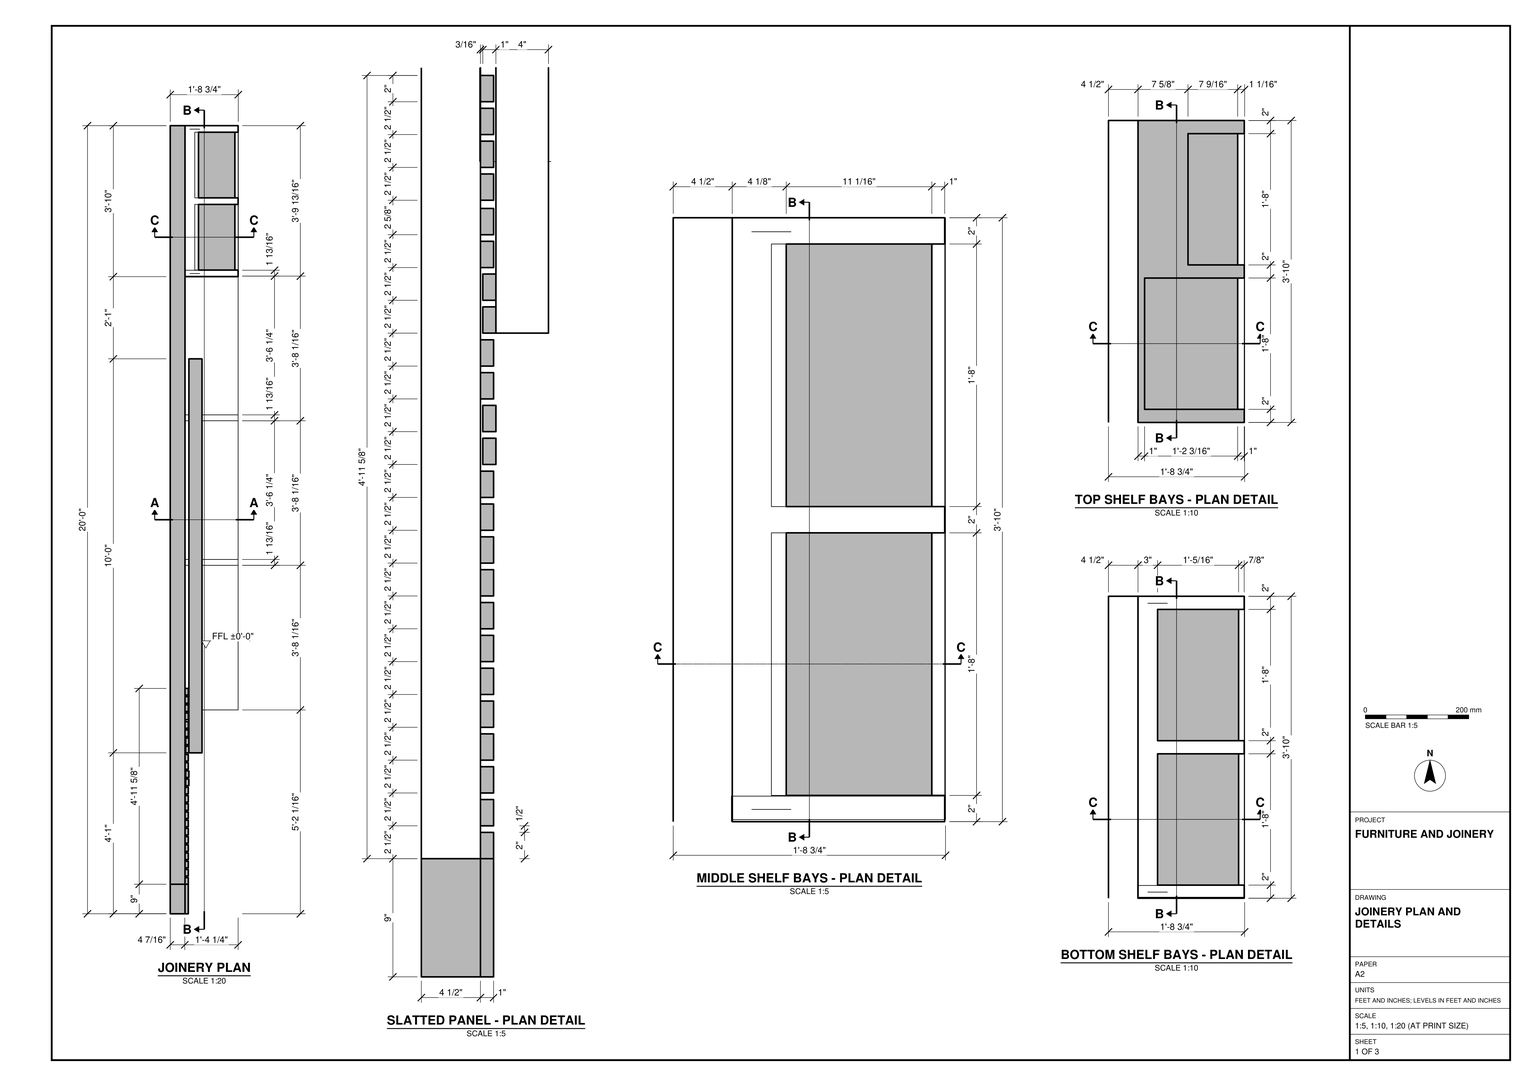
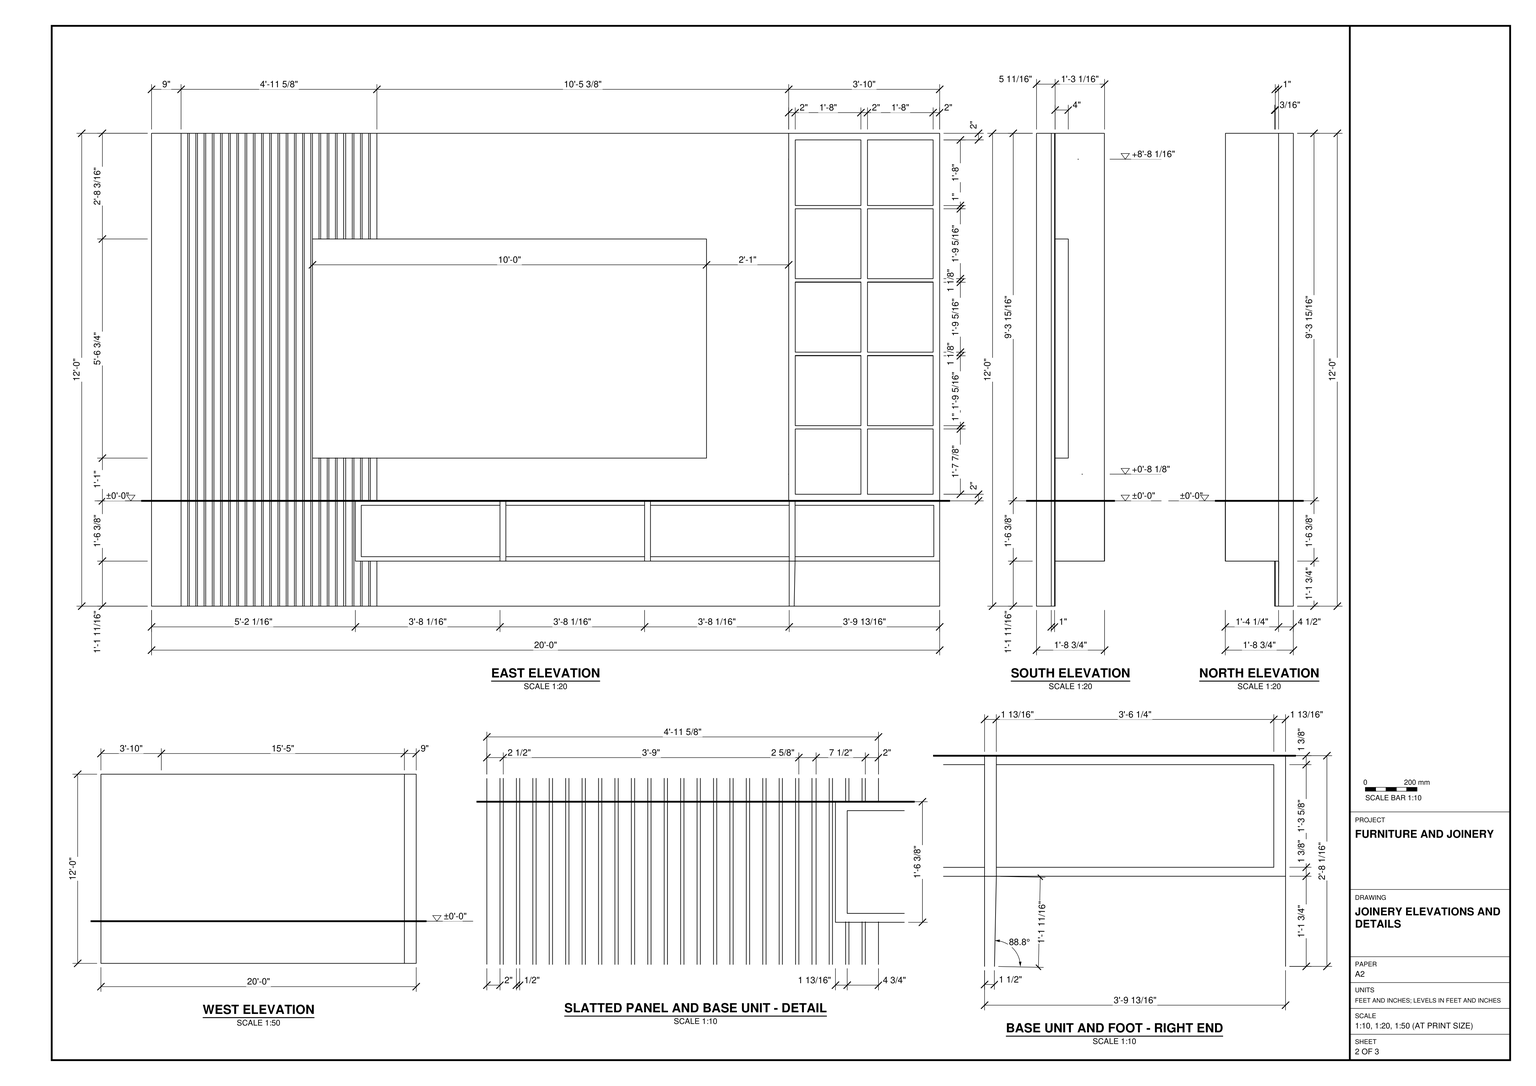
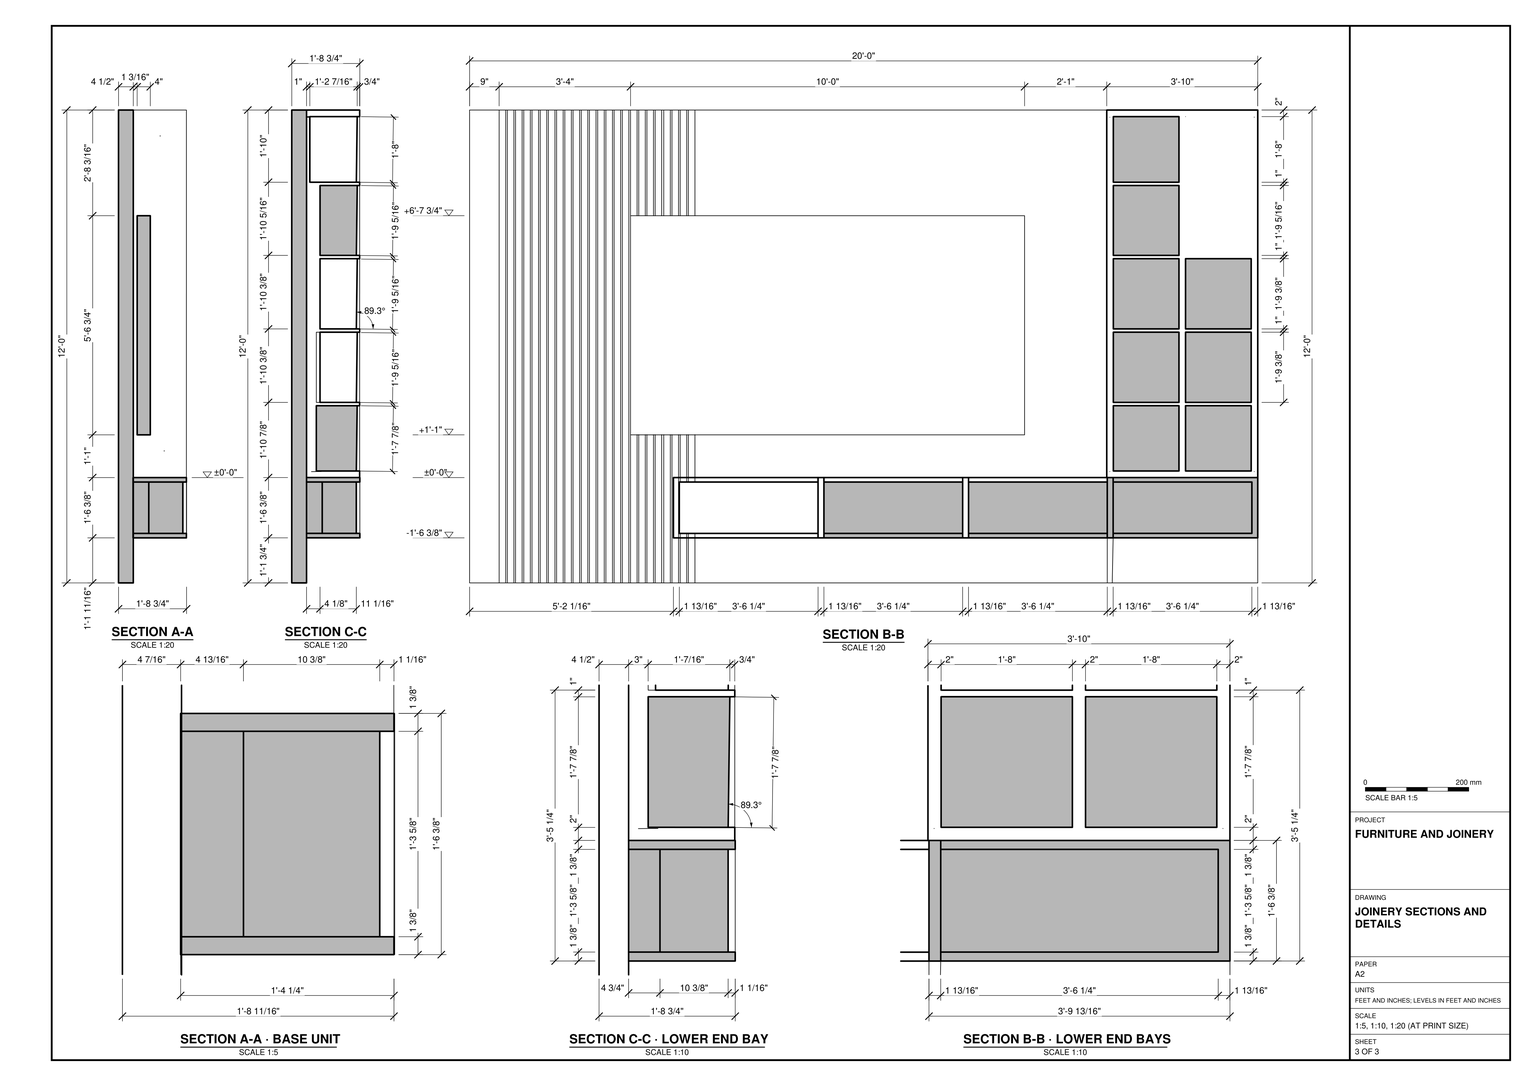
Build the wall unit in SketchUp from task_files/diagram_01.pdf. Work in feet and inches. The unit is 20'-0" long along Y, 1'-8 3/4" deep along X and 12'-0" high along Z. Use the finished-floor datum of ±0'-0" shown in the sections: it aligns with the top of the base unit, not the bottom of the backing panel.

Use the east elevation to lay out the front. Model the full-height backing panel with a plain margin at the left, followed by a field of projecting vertical slats. Set the large rectangular panel in front of the backing so that its left end overlaps the slats. Leave the drawn gap between its right end and the shelving. At the right, form the two-column shelf tower and use the top, middle and bottom bay plans to set the depths of the bay parts rather than relying on the front view alone.

Run the four-compartment base unit from within the slatted area to the right end, with the narrow support beneath it as detailed. Model the board thicknesses, dividers and projections shown in the sections. Keep distinct joinery assemblies in separate groups or components and use components for repeated parts. Any decor or loose items may use suitable library components. Save one SketchUp model as output_files/slatted_wall_unit_with_shelving_and_base_storage.skp.

# SketchUp Ruby script. Lengths in inches.
U = 1.inch
M = Sketchup.active_model
def pt(a) = Geom::Point3d.new(a.map { |v| v * U })
def face(e, loops, mat)
  f = e.add_face(loops[0].map { |a| pt(a) })
  loops[1..].each { |l| e.add_face(l.map { |a| pt(a) }).erase! }
  f.material = f.back_material = mat if mat
  f
end
# faces: each face lists its corners as indices into pts; further lists are holes
def faces(e, pts, list, mat = nil) = list.each { |f| face(e, (f[0].is_a?(Array) ? f : [f]).map { |l| l.map { |i| pts[i] } }, mat) }
# xy, xz, yz: faces in a plane at the given z, y or x. An outline is a flat list of corners, or four numbers for a rectangle; further outlines are holes
def ring(l) = l.size == 4 ? [[l[0], l[1]], [l[2], l[1]], [l[2], l[3]], [l[0], l[3]]] : l.each_slice(2).to_a
def flat(e, list, mat, &to3) = list.each { |f| face(e, (f[0].is_a?(Array) ? f : [f]).map { |l| ring(l).map { |u, v| to3.(u, v) } }, mat) }
def xy(e, z, list, mat = nil) = flat(e, list, mat) { |x, y| [x, y, z] }
def xz(e, y, list, mat = nil) = flat(e, list, mat) { |x, z| [x, y, z] }
def yz(e, x, list, mat = nil) = flat(e, list, mat) { |y, z| [x, y, z] }
def lines(e, pts, list) = list.each { |a, b| e.add_line(pt(pts[a]), pt(pts[b])) }
# prism: a flat outline (further loops are holes) pulled along v
def prism(e, loops, v, mat = nil)
  f = face(e, loops, mat); d = Geom::Vector3d.new(v.map { |x| x * U })
  f.pushpull(f.normal.samedirection?(d) ? d.length : -d.length)
end
def box(e, o, s, mat = nil) = prism(e, [[o, [o[0] + s[0], o[1], o[2]], [o[0] + s[0], o[1] + s[1], o[2]], [o[0], o[1] + s[1], o[2]]]], [0, 0, s[2]], mat)
def at(x, y, z, deg = 0) = Geom::Transformation.translation(pt([x, y, z])) * Geom::Transformation.rotation(ORIGIN, Z_AXIS, deg.degrees)
def axes(o, x, y, z) = Geom::Transformation.new([*x, 0, *y, 0, *z, 0, *pt(o).to_a, 1])
def part(name) = M.definitions.add(name)
# library, detail: a bought-in or finely detailed component or shape, given as its bounding box
def library(name, o, s) = part(name).tap { |d| box(d.entities, o, s) }
def detail(e, o, s) = box(e.add_group.entities, o, s)
def put(e, d, t, mat = nil) = e.add_instance(d, t).tap { |i| i.material = mat if mat }
def group(e, t, mat = nil) = e.add_group.tap { |g| g.transformation = t; g.material = mat if mat }.entities
root = M.entities
M.materials.add("[0099_LightSteelBlue]").color = [176, 196, 222]
M.materials.add("[Color E08]").color = [102, 102, 0]
M.materials.add("[Stone Brushed Khaki]").color = [226, 197, 133]
M.materials.add("[Stone Marble]").color = [143, 138, 136]
M.materials.add("[Translucent Glass Blue]").color = [100, 149, 237]
M.materials["[Translucent Glass Blue]"].alpha = 0.5
M.materials.add("[Wood Cherry Original]").color = [152, 86, 42]
M.materials.add("[Wood Plywood Knots]").color = [137, 122, 41]
c1 = part("Vertical slat")
box(c1.entities,[0,0,0],[1,2,144])
c2 = part("Wall slat assembly")
put(c2.entities,c1,at(0.41,0,0),"[Wood Cherry Original]")
put(c2.entities,c1,at(0.41,2.5,0),"[Wood Cherry Original]")
c3 = part("Base storage unit")
xy(c3.entities,-1.48,[[-2.48,29.14,11.52,54.74]],"[Wood Plywood Knots]")
xy(c3.entities,-0.48,[[-2.48,30.14,1.65,53.74],[1.65,30.14,10.59,53.74]])
xy(c3.entities,-0.48,[[10.59,30.14,11.52,53.74]],"[Wood Plywood Knots]")
xy(c3.entities,11.02,[[-2.48,30.14,1.65,53.74],[1.65,30.14,10.59,53.74]])
xy(c3.entities,11.02,[[10.59,30.14,11.52,53.74]],"[Wood Plywood Knots]")
xy(c3.entities,12.02,[[-2.48,29.14,11.52,54.74]],"[Wood Plywood Knots]")
xz(c3.entities,29.14,[[-2.48,-1.48,11.52,12.02]],"[Wood Plywood Knots]")
xz(c3.entities,30.14,[[-2.48,-0.48,1.65,11.02],[1.65,-0.48,10.59,11.02]])
xz(c3.entities,30.14,[[10.59,-0.48,11.52,11.02]],"[Wood Plywood Knots]")
xz(c3.entities,53.74,[[-2.48,-0.48,1.65,11.02],[1.65,-0.48,10.59,11.02]])
xz(c3.entities,53.74,[[10.59,-0.48,11.52,11.02]],"[Wood Plywood Knots]")
xz(c3.entities,54.74,[[-2.48,-1.48,11.52,12.02]],"[Wood Plywood Knots]")
yz(c3.entities,-2.48,[[[29.14,-1.48,54.74,12.02],[30.14,-0.48,53.74,11.02]],[30.14,-0.48,53.74,11.02]],"[Wood Plywood Knots]")
yz(c3.entities,1.65,[[30.14,-0.48,53.74,11.02]])
yz(c3.entities,10.59,[[30.14,-0.48,53.74,11.02]],"[Translucent Glass Blue]")
yz(c3.entities,11.52,[[[29.14,-1.48,54.74,12.02],[30.14,-0.48,53.74,11.02]]],"[Wood Plywood Knots]")
xy(root,100.426,[[19.659,196.022,20.663,216.011],[19.659,218.011,20.663,238]],"[Wood Plywood Knots]")
xy(root,122.809,[[19.661,196.022,20.665,216.011],[19.661,218.011,20.665,238]],"[Wood Plywood Knots]")
xy(root,145.192,[[19.663,196.022,20.667,216.011],[19.663,218.011,20.667,238]],"[Wood Plywood Knots]")
xy(root,166.476,[[19.939,196.022,20.669,216.011],[19.939,218.011,20.669,238]],"[Wood Plywood Knots]")
xy(root,187.458,[[12.109,218.011,19.92,238]],"[Wood Plywood Knots]")
xz(root,194.022,[[20.661,77.543,20.672,189.457,4.5,189.459,4.49,77.545]],"[Wood Plywood Knots]")
xz(root,196.022,[[19.655,79.537,7.474,79.545,7.476,99.427,19.912,99.42],[19.655,79.537,19.912,99.42,20.663,99.426,20.661,79.543],[19.659,100.426,8.601,100.427,8.603,121.81,20.665,121.809,20.663,100.426],[19.661,122.809,8.603,122.81,8.605,144.193,20.667,144.192,20.665,122.809],[19.663,145.192,8.605,145.193,8.607,166.477,19.939,166.476],
  [19.663,145.192,19.939,166.476,20.669,166.476,20.667,145.192],[19.662,167.476,5.498,167.478,5.5,187.459,19.92,187.458],[19.662,167.476,19.92,187.458,20.671,187.457,20.67,167.476]],"[Wood Plywood Knots]")
xz(root,216.011,[[19.655,79.537,19.912,99.42,7.476,99.427,7.474,79.545],[19.655,79.537,20.661,79.543,20.663,99.426,19.912,99.42],[19.659,100.426,20.663,100.426,20.665,121.809,8.603,121.81,8.601,100.427],[19.661,122.809,20.665,122.809,20.667,144.192,8.605,144.193,8.603,122.81],[19.663,145.192,19.939,166.476,8.607,166.477,8.605,145.193],
  [19.663,145.192,20.667,145.192,20.669,166.476,19.939,166.476],[19.662,167.476,19.92,187.458,5.5,187.459,5.498,167.478],[19.662,167.476,20.67,167.476,20.671,187.457,19.92,187.458]],"[Wood Plywood Knots]")
xz(root,218.011,[[19.655,79.543,7.474,79.545,7.476,99.427,20.663,99.426,20.661,79.543],[19.659,100.426,7.476,100.427,7.478,121.81,20.665,121.809,20.663,100.426],[19.661,122.809,8.603,122.81,8.605,144.193,20.667,144.192,20.665,122.809],[19.663,145.192,11.792,145.193,11.794,166.477,19.939,166.476],[19.663,145.192,19.939,166.476,20.669,166.476,20.667,145.192],
  [19.662,167.476,12.107,167.477,12.109,187.458,19.92,187.458],[19.662,167.476,19.92,187.458,20.671,187.457,20.67,167.476]],"[Wood Plywood Knots]")
xz(root,238,[[19.655,79.543,20.661,79.543,20.663,99.426,7.476,99.427,7.474,79.545],[19.659,100.426,20.663,100.426,20.665,121.809,7.478,121.81,7.476,100.427],[19.661,122.809,20.665,122.809,20.667,144.192,8.605,144.193,8.603,122.81],[19.663,145.192,19.939,166.476,11.794,166.477,11.792,145.193],[19.663,145.192,20.667,145.192,20.669,166.476,19.939,166.476],
  [19.662,167.476,19.92,187.458,12.109,187.458,12.107,167.477],[19.662,167.476,20.67,167.476,20.671,187.457,19.92,187.458]],"[Wood Plywood Knots]")
xz(root,240,[[20.661,77.543,4.49,77.545,4.5,189.459,20.672,189.457,20.67,167.075]],"[Wood Plywood Knots]")
p = [[4.5,240,189.459],[4.49,240,77.545],[4.49,194.022,77.545],[4.5,194.022,189.459],[20.661,240,77.543],[20.661,194.022,77.543],
  [20.672,240,189.457],[20.672,194.022,189.457],[20.67,240,167.075],[20.663,196.022,100.426],[20.665,196.022,121.809],[20.665,216.011,121.809],
  [20.663,216.011,100.426],[20.667,196.022,144.192],[20.667,216.011,144.192],[20.665,216.011,122.809],[20.665,196.022,122.809],[20.665,218.011,121.809],
  [20.665,238,121.809],[20.663,238,100.426],[20.663,218.011,100.426],[20.667,218.011,144.192],[20.667,238,144.192],[20.665,238,122.809],
  [20.665,218.011,122.809],[20.669,238,166.476],[20.667,238,145.192],[20.667,218.011,145.192],[20.669,218.011,166.476],[20.669,196.022,166.476],
  [20.669,216.011,166.476],[20.667,216.011,145.192],[20.667,196.022,145.192],[20.67,218.011,167.476],[20.671,218.011,187.457],[20.671,238,187.457],
  [20.67,238,167.476],[20.671,216.011,187.457],[20.67,216.011,167.476],[20.67,196.022,167.476],[20.671,196.022,187.457],[20.661,216.011,79.543],
  [20.661,196.022,79.543],[20.663,196.022,99.426],[20.663,216.011,99.426],[20.663,218.011,99.426],[20.663,238,99.426],[20.661,238,79.543],
  [20.661,218.011,79.543],[7.474,216.011,79.545],[7.476,216.011,99.427],[7.476,196.022,99.427],[7.474,196.022,79.545],[19.655,196.022,79.537],
  [19.655,216.011,79.537],[19.912,216.011,99.42],[19.912,196.022,99.42],[7.474,218.011,79.545],[7.474,238,79.545],[7.476,238,99.427],
  [7.476,218.011,99.427],[19.655,238,79.543],[19.655,218.011,79.543],[19.912,238,99.42],[19.912,218.011,99.42],[19.655,218.011,79.537],
  [19.655,238,79.537],[8.603,196.022,121.81],[8.601,196.022,100.427],[8.601,216.011,100.427],[8.603,216.011,121.81],[19.659,196.022,100.426],
  [19.659,216.011,100.426],[19.935,196.022,121.711],[19.935,216.011,121.711],[7.478,218.011,121.81],[7.476,218.011,100.427],[7.476,238,100.427],
  [7.478,238,121.81],[19.659,218.011,100.426],[19.659,238,100.426],[19.935,218.011,121.711],[19.935,238,121.711],[8.605,196.022,144.193],
  [8.603,196.022,122.81],[8.603,216.011,122.81],[8.605,216.011,144.193],[19.661,196.022,122.809],[19.661,216.011,122.809],[19.937,196.022,144.094],
  [19.937,216.011,144.094],[8.605,218.011,144.193],[8.603,218.011,122.81],[8.603,238,122.81],[8.605,238,144.193],[19.661,218.011,122.809],
  [19.661,238,122.809],[19.937,218.011,144.094],[19.937,238,144.094],[8.607,196.022,166.477],[8.605,196.022,145.193],[8.605,216.011,145.193],
  [8.607,216.011,166.477],[19.663,196.022,145.192],[19.663,216.011,145.192],[19.939,196.022,166.476],[19.939,216.011,166.476],[11.794,218.011,166.477],
  [11.792,218.011,145.193],[11.792,238,145.193],[11.794,238,166.477],[19.663,218.011,145.192],[19.663,238,145.192],[19.939,218.011,166.476],
  [19.939,238,166.476],[5.5,216.011,187.459],[5.5,196.022,187.459],[5.498,196.022,167.478],[5.498,216.011,167.478],[19.662,216.011,167.476],
  [19.662,196.022,167.476],[19.92,216.011,187.458],[19.662,216.011,167.47],[19.662,196.022,167.47],[19.92,196.022,187.458],[12.109,218.011,187.458],
  [12.107,218.011,167.477],[12.107,238,167.477],[12.109,238,187.458],[19.662,238,167.476],[19.662,218.011,167.476],[19.92,238,187.458],
  [19.662,238,167.47],[19.662,218.011,167.47],[19.92,218.011,187.458],[4.5,216.011,187.459],[5.982,194.954,79.346],[8.965,194.954,79.385],
  [4.595,194.954,187.251],[5.595,194.954,187.264],[5.982,238.932,79.346],[8.965,238.932,79.385],[12.781,193.954,181.572],[12.595,193.954,181.57],
  [13.827,193.954,85.649],[14.013,193.954,85.651],[4.595,238.932,187.251],[12.204,238.932,187.349],[4.5,218.011,187.459],[4.49,194.176,59.185],
  [4.5,194.176,45.459],[4.43,195.966,59.175],[4.5,195.684,45.459],[4.5,195.966,59.175]]
faces(root,p,[[0,1,2,3],[2,1,4,5]])
faces(root,p,[[[6,7,5,4,8],[9,10,11,12],[13,14,15,16],[17,18,19,20],[21,22,23,24],[25,26,27,28],[29,30,31,32],[33,34,35,36],[37,38,39,40],[41,42,43,44],[45,46,47,48]],[49,50,51,52],[52,53,54,49],[41,54,53,42],[57,58,59,60],[48,47,61,58,57,62],[50,55,56,51],[43,56,55,44],
  [46,45,60,59],[67,68,69,70],[68,71,72,69],[75,76,77,78],[76,79,80,77],[11,10,67,70],[18,17,75,78],[83,84,85,86],
  [84,87,88,85],[91,92,93,94],[92,95,96,93],[14,13,83,86],[22,21,91,94],[99,100,101,102],[100,103,104,101],[107,108,109,110],
  [108,111,112,109],[102,106,105,99],[110,114,113,107],[115,116,117,118],[39,38,119,118,117,120],[125,126,127,128],[33,36,129,127,126,130],[115,121,124,116],
  [40,124,121,37],[34,134,131,35],[0,3,7,6]],"[Wood Plywood Knots]")
faces(root,p,[[55,56,53,54],[63,64,62,65,66,61],[71,73,74,72],[79,81,82,80],[87,89,90,88],[95,97,98,96],[103,105,106,104],[111,113,114,112],
  [121,119,122,123,120,124],[131,129,132,133,130,134]],"[Translucent Glass Blue]")
lines(root,p,[[135,115],[136,137],[138,139],[140,141],[142,143],[144,145],[146,147],[148,125],[149,150],[151,152],[152,153]])
put(root,c2,at(4.09,9,45.46),"[Wood Cherry Original]")
put(root,c2,at(4.09,14,45.46),"[Wood Cherry Original]")
put(root,c2,at(4.09,19,45.46),"[Wood Cherry Original]")
put(root,c2,at(4.09,24,45.46),"[Wood Cherry Original]")
put(root,c2,at(4.09,29,45.46),"[Wood Cherry Original]")
put(root,c2,at(4.09,34,45.46),"[Wood Cherry Original]")
put(root,c2,at(4.27,39.01,45.46),"[Wood Cherry Original]")
put(root,c2,at(4.09,44,45.46),"[Wood Cherry Original]")
put(root,c2,at(4.27,49.01,45.46),"[Wood Cherry Original]")
put(root,c2,at(4.09,54,45.46),"[Wood Cherry Original]")
put(root,c3,axes([7.3,9.91,61.19],[1.16,0,0],[0,1.79,0],[0,0,1.36]))
put(root,c3,axes([7.3,53.94,61.19],[1.16,0,0],[0,1.79,0],[0,0,1.36]))
put(root,c2,at(4.09,59.125,45.46),"[Wood Cherry Original]")
put(root,c2,at(4.09,64.125,45.46),"[Wood Cherry Original]")
put(root,c3,axes([7.3,97.98,61.19],[1.16,0,0],[0,1.79,0],[0,0,1.36]))
put(root,c3,axes([7.36,142.01,61.2],[1.16,0,0],[0,1.79,0],[0,0,1.36]))
g1 = group(root,at(0,0,45.46))
xy(g1,0,[[0,0,4.5,240]])
xy(g1,144,[[0,0,4.5,240]])
xz(g1,0,[[0,0,4.5,144]])
xz(g1,240,[[0,0,4.5,144]])
yz(g1,0,[[0,0,240,144]])
yz(g1,4.5,[[0,0,240,144]],"[Stone Brushed Khaki]")
g2 = group(root,at(0,-9,45.46),"[0099_LightSteelBlue]")
xy(g2,0,[[0,9,5.5,18]])
xy(g2,144,[[0,9,5.5,18]])
xz(g2,9,[[0,0,5.5,144]])
xz(g2,18,[[0,0,5.5,144]])
yz(g2,0,[[9,0,18,144]])
yz(g2,5.5,[[9,0,18,144]],"[Stone Marble]")
g3 = group(root,at(5.68,31.01,90.55),"[Color E08]")
box(g3,[0,18,0],[4,119.99,66.73],"[Color E08]")
